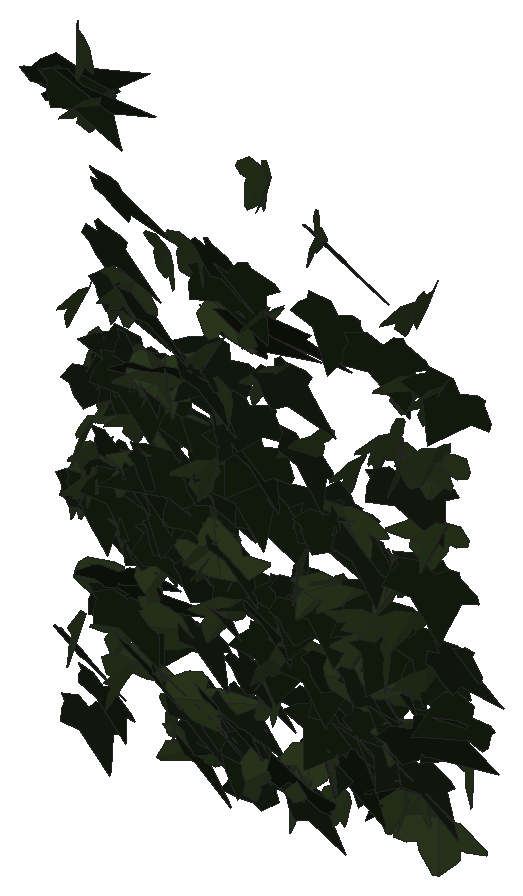
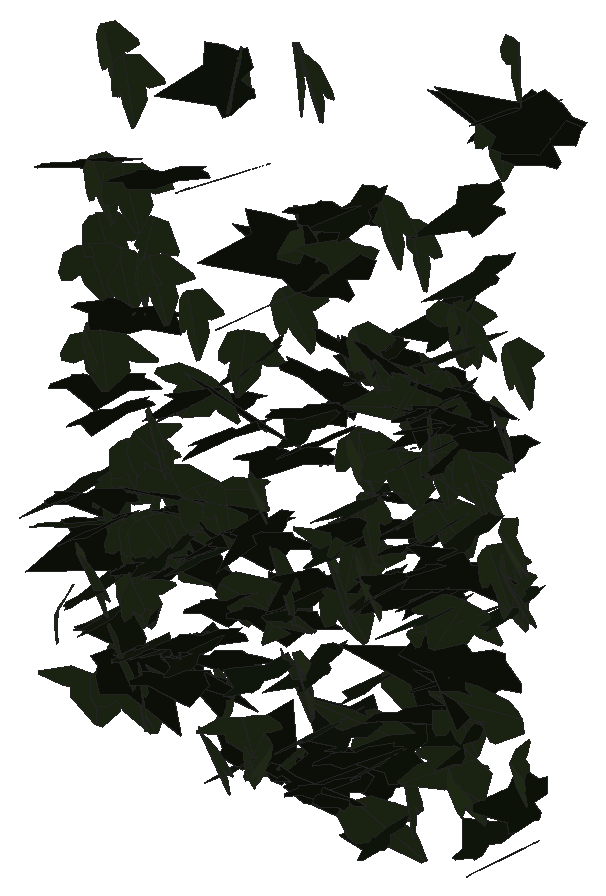
# SketchUp Ruby script. Lengths in millimetres.
U = 1.mm
M = Sketchup.active_model
def pt(a) = Geom::Point3d.new(a.map { |v| v * U })
def face(e, loops, mat)
  f = e.add_face(loops[0].map { |a| pt(a) })
  loops[1..].each { |l| e.add_face(l.map { |a| pt(a) }).erase! }
  f.material = f.back_material = mat if mat
  f
end
# faces: each face lists its corners as indices into pts; further lists are holes
def faces(e, pts, list, mat = nil) = list.each { |f| face(e, (f[0].is_a?(Array) ? f : [f]).map { |l| l.map { |i| pts[i] } }, mat) }
# xy, xz, yz: faces in a plane at the given z, y or x. An outline is a flat list of corners, or four numbers for a rectangle; further outlines are holes
def ring(l) = l.size == 4 ? [[l[0], l[1]], [l[2], l[1]], [l[2], l[3]], [l[0], l[3]]] : l.each_slice(2).to_a
def flat(e, list, mat, &to3) = list.each { |f| face(e, (f[0].is_a?(Array) ? f : [f]).map { |l| ring(l).map { |u, v| to3.(u, v) } }, mat) }
def xy(e, z, list, mat = nil) = flat(e, list, mat) { |x, y| [x, y, z] }
def xz(e, y, list, mat = nil) = flat(e, list, mat) { |x, z| [x, y, z] }
def yz(e, x, list, mat = nil) = flat(e, list, mat) { |y, z| [x, y, z] }
def lines(e, pts, list) = list.each { |a, b| e.add_line(pt(pts[a]), pt(pts[b])) }
# prism: a flat outline (further loops are holes) pulled along v
def prism(e, loops, v, mat = nil)
  f = face(e, loops, mat); d = Geom::Vector3d.new(v.map { |x| x * U })
  f.pushpull(f.normal.samedirection?(d) ? d.length : -d.length)
end
def box(e, o, s, mat = nil) = prism(e, [[o, [o[0] + s[0], o[1], o[2]], [o[0] + s[0], o[1] + s[1], o[2]], [o[0], o[1] + s[1], o[2]]]], [0, 0, s[2]], mat)
def at(x, y, z, deg = 0) = Geom::Transformation.translation(pt([x, y, z])) * Geom::Transformation.rotation(ORIGIN, Z_AXIS, deg.degrees)
def axes(o, x, y, z) = Geom::Transformation.new([*x, 0, *y, 0, *z, 0, *pt(o).to_a, 1])
def part(name) = M.definitions.add(name)
# library, detail: a bought-in or finely detailed component or shape, given as its bounding box
def library(name, o, s) = part(name).tap { |d| box(d.entities, o, s) }
def detail(e, o, s) = box(e.add_group.entities, o, s)
def put(e, d, t, mat = nil) = e.add_instance(d, t).tap { |i| i.material = mat if mat }
def group(e, t, mat = nil) = e.add_group.tap { |g| g.transformation = t; g.material = mat if mat }.entities
root = M.entities
M.materials.add("efeu1").color = [18, 25, 13]
M.materials.add("efeu2").color = [43, 57, 29]
c1 = part("ivyleaf_9")
p = [[39.1,54.8,31.7],[34.5,51.8,30.2],[-5.3,25.2,17.3],[-17.9,28.3,20.9],[-21.6,21.7,17],[-20.2,4.3,5.3],
  [-22.9,-0.3,2.5],[-17.1,-4,-0.6],[-2,-2.1,-1.2],[-0.7,-15.4,-10.1],[16.6,-22.3,-16.7],[21.1,-15.1,-12.5],
  [32.7,-10.7,-11],[46.1,-1.8,-6.6],[30.8,11.2,3.8]]
faces(c1.entities,p,[[0,1,2,3,4,5,6,7,8,9,10,11,12,13,14]],"efeu1")
c2 = part("ivyleaf_10")
p = [[0,12.8,-0.8],[-1.5,51.3,-10.9],[-4.9,51,-11.6],[-13.6,26.5,-7.3],[-13.2,15.9,-4.6],[-21.1,19.3,-7.2],
  [-29.5,16.3,-8.3],[-29.2,8.3,-6.2],[-19.7,-9.8,0.5],[-7.6,-13,4],[1,-12.2,5.8],[-0.4,51.1,-11.1],
  [-1.5,51.1,-10.9],[1,-12.4,5.9],[16.9,-12.4,3.5],[35.1,9.1,-5.1],[35,12.9,-6.1],[20.5,16.4,-4.9],
  [15.8,15,-3.8],[15.3,27.6,-7.1],[12.8,31.3,-7.8]]
faces(c2.entities,p,[[0,1,2,3,4,5,6,7,8,9,10],[11,12,0,13,14,15,16,17,18,19,20]],"efeu2")
put(root,c1,axes([1990.1,917.2,1718.9],[1.12387,-0.63107,0.1221],[0.14327,-0.09676,-0.8642],[1.21491,0.59519,-0.01104]))
put(root,c2,axes([2008.9,912.7,1745.6],[0.40299,-0.65276,0.62987],[0.55976,-0.56245,-0.68177],[1.63313,0.35386,0.07825]))
put(root,c2,axes([2015,919.8,1993.4],[0.61387,-0.7633,0.37634],[0.25359,-0.3522,-0.82855],[1.59972,0.34874,-0.01307]))
put(root,c2,axes([2011.3,925.5,1957.4],[0.80255,-0.66619,0.47453],[0.51309,-0.39084,-0.78827],[1.46967,0.50024,0.01607]))
put(root,c2,axes([2030,891.6,2498.3],[-0.97213,0.83488,0.13187],[-0.54697,-0.02666,-0.94446],[-1.51279,-0.52686,0.25675]))
put(root,c2,axes([2026.4,897.1,2176.3],[0.05785,-0.94512,0.06097],[0.02216,-0.06063,-0.94556],[1.80235,0.03108,0.00967]))
put(root,c1,axes([1991.5,894.9,2427],[0.1501,0.02213,0.98086],[1.85842,0.09385,-0.08063],[-0.18145,0.97954,-0.01443]))
put(root,c2,axes([2028,924.3,1970.1],[-0.2482,-0.88121,0.04249],[-0.01566,-0.04174,-0.89081],[1.679,-0.13066,-0.00203]))
put(root,c2,axes([2027.2,905.9,1933.9],[0.05965,-0.89479,0.23589],[0.10716,-0.23374,-0.89413],[1.75789,0.04461,0.0465]))
put(root,c2,axes([2017.5,913.4,1936.6],[1.16603,-0.58752,0.35337],[0.48398,-0.24537,-0.84885],[1.21177,0.66335,-0.00101]))
put(root,c1,axes([2008.1,914.5,1921.8],[0.66197,-0.86169,-0.09061],[-0.04948,0.08722,-0.9292],[1.64827,0.34869,0.0085]))
put(root,c1,axes([1989.1,894.6,2420.1],[0.75999,-0.14629,0.88705],[1.58589,-0.30414,-0.42527],[0.64232,0.92402,0.00046]))
put(root,c2,axes([2039.3,905.8,2111.2],[0.62311,-0.87046,-0.11063],[-0.05092,0.10813,-0.92991],[1.66921,0.32824,0.01293]))
put(root,c1,axes([2019.2,895.9,2444.3],[0.1992,-0.87795,-0.42366],[0.07153,0.42941,-0.88058],[1.8539,0.07776,0.0795]))
put(root,c2,axes([2044.4,898.7,2422.2],[-0.51083,-0.92636,-0.14907],[0.02925,0.15069,-0.96408],[1.78548,-0.2675,-0.02686]))
put(root,c1,axes([2027.1,909.1,1644.1],[0.07903,-0.88048,0.00723],[-0.00064,-0.00725,-0.88146],[1.67579,0.04152,-0.00068]))
put(root,c1,axes([2029.3,918.9,1916.4],[-0.17209,-0.89353,0.13845],[0.07065,-0.14269,-0.89667],[1.71942,-0.08357,0.0507]))
put(root,c2,axes([2020.4,924.2,1807],[-0.35173,-0.00066,-0.86106],[1.59723,-0.19716,-0.17998],[-0.36662,-0.85832,0.042]))
put(root,c1,axes([2033,927.2,1665],[0.10984,-0.76984,0.47996],[0.25295,-0.46857,-0.76755],[1.70797,0.1189,0.08281]))
put(root,c2,axes([2060,916.5,2061.2],[-0.44307,-0.89746,-0.00374],[-0.00659,0.00476,-0.92716],[1.70805,-0.23278,-0.00455]))
put(root,c1,axes([2041.2,899.1,2083.9],[0.33132,-0.44315,-0.83753],[0.01285,0.85211,-0.44946],[1.80332,0.07535,0.15708]))
put(root,c2,axes([2078.8,909.2,2200],[-1.61919,0.44371,-0.02949],[-0.18807,-0.2507,-0.92138],[-0.82517,-0.81353,0.26786]))
put(root,c1,axes([2052,898.5,2256.9],[1.02908,-0.75368,-0.2417],[-0.10045,0.25773,-0.92174],[1.503,0.53326,0.10388]))
put(root,c2,axes([2088.4,918.4,2049.3],[1.45985,0.05981,-0.52265],[-1.00038,0.04982,-0.76572],[-0.04043,0.92685,0.07488]))
put(root,c2,axes([2079.2,912.6,1708.9],[0.12496,-0.88374,0.32845],[0.03978,-0.3278,-0.88617],[1.79391,0.06883,-0.00323]))
put(root,c1,axes([2077.4,899.4,1839.3],[1.22739,0.6361,-0.27839],[-0.36762,-0.20059,-0.90581],[-1.26933,0.67318,-0.00685]))
put(root,c1,axes([2056.2,921.6,2188.5],[0.59629,-0.83809,-0.26319],[0.10399,0.29748,-0.88224],[1.66862,0.28096,0.14903]))
put(root,c1,axes([2057.7,918.5,1983.1],[0.44094,-0.90044,0.27415],[0.12071,-0.26676,-0.92975],[1.78731,0.24016,-0.00484]))
put(root,c2,axes([2085.6,901.3,2200.9],[-0.10632,-0.94317,0.10208],[0.04003,-0.10346,-0.94444],[1.80508,-0.05326,0.02696]))
put(root,c1,axes([2059.8,923.5,1952.1],[-0.45177,-0.37457,-0.79739],[1.02127,0.59349,-0.43853],[1.32977,-0.58305,0.06589]))
put(root,c1,axes([2060.2,893,2326.8],[1.43127,-0.51566,-0.29418],[-0.21832,0.33961,-0.88854],[1.10858,0.73264,0.20482]))
put(root,c2,axes([2089.7,903,1778.1],[-0.70668,-0.78897,0.20128],[-0.08513,-0.20112,-0.87086],[1.54732,-0.3714,0.04401]))
put(root,c1,axes([2080.2,917.8,1940.1],[-0.78015,-0.78959,-0.16269],[0.17537,0.13543,-0.88945],[1.52427,-0.41971,0.01906]))
put(root,c2,axes([2083.5,911.3,1890.1],[-1.60821,-0.14706,-0.20845],[0.40193,0.00133,-0.85703],[0.27234,-0.87033,0.03391]))
put(root,c1,axes([2098.9,911.3,2118.6],[-1.63713,-0.36913,-0.1268],[0.22874,0.04145,-0.93601],[0.70673,-0.8685,0.00922]))
put(root,c2,axes([2076.9,913.2,1727.6],[-0.92159,-0.27206,-0.68845],[1.16217,0.31822,-0.55526],[0.79638,-0.77921,0.01361]))
put(root,c2,axes([2105.3,907.5,1984.7],[-0.88953,-0.68114,0.40284],[-0.18018,-0.41637,-0.81385],[1.49527,-0.45538,0.14158]))
put(root,c1,axes([2080.3,911.9,1803.8],[-0.86853,-0.30959,-0.73877],[1.21639,0.37179,-0.55061],[0.91895,-0.78473,0.03059]))
put(root,c2,axes([2104.7,904.6,2052],[-0.53625,-0.95589,-0.13853],[0.07205,0.13326,-0.99655],[1.83685,-0.28429,-0.00135]))
put(root,c1,axes([2089.7,899.6,1806.1],[-0.17767,-0.79826,-0.4047],[0.1152,0.40033,-0.80361],[1.69943,-0.11059,0.01216]))
put(root,c1,axes([2093.4,920.8,2113.9],[0.08019,-0.89919,0.24159],[-0.02149,-0.24232,-0.89991],[1.7719,0.03775,-0.02185]))
put(root,c1,axes([2081.4,908.5,1747.1],[0.80924,-0.75365,0.41974],[0.38074,-0.36905,-0.8653],[1.59704,0.46987,-0.00639]))
put(root,c1,axes([2099.9,907.2,2098.7],[-0.54646,-0.94966,-0.20046],[0.14069,0.18705,-0.99198],[1.84186,-0.29604,0.0163]))
put(root,c1,axes([2127.4,917.6,2091.2],[-1.56948,-0.3673,0.14155],[-0.244,-0.06006,-0.90275],[0.70831,-0.83455,0.00267]))
put(root,c2,axes([2146.3,906.3,1791.5],[-0.60734,-0.0873,0.93419],[-1.65812,-0.33871,-0.32926],[0.66286,-0.92727,0.03232]))
put(root,c2,axes([2114.8,911.8,2094.9],[0.39495,-0.8249,-0.38584],[0.08041,0.40402,-0.84105],[1.73133,0.16941,0.12708]))
put(root,c1,axes([2099.4,919.5,1907.4],[0.14005,-0.87197,-0.23761],[-0.04436,0.23648,-0.87507],[1.71948,0.07712,-0.00322]))
put(root,c1,axes([2095.4,911.5,1888.2],[0.86165,-0.65292,-0.42802],[-0.10478,0.46685,-0.77039],[1.48215,0.41258,0.19437]))
put(root,c1,axes([2101.7,917.7,1972],[0.23204,-0.89795,0.0866],[-0.00199,-0.08752,-0.9061],[1.71691,0.12126,-0.01276]))
put(root,c1,axes([2094.5,901.3,2194.3],[1.04166,-0.78648,0.00423],[0.00467,-0.00345,-0.95818],[1.49684,0.54733,0.00004]))
put(root,c1,axes([2103.8,930.9,2061.6],[0.09179,-0.91788,-0.03431],[-0.00004,0.03436,-0.91915],[1.74814,0.0482,0.00178]))
put(root,c1,axes([2100,906.9,2080.8],[0.17781,-0.78896,-0.46319],[0.28795,0.47251,-0.77432],[1.71722,0.00246,0.1778]))
put(root,c2,axes([2124,890.9,1845.4],[0.21699,0.3029,-0.87536],[0.375,0.85385,0.32112],[1.72256,-0.22404,0.04036]))
put(root,c1,axes([2094.2,904.8,1813],[0.73125,0.39717,-0.69678],[0.93475,0.49428,0.55257],[1.20673,-0.62355,-0.0058]))
put(root,c2,axes([2099.6,903.5,2115.7],[0.98585,-0.27331,0.72979],[1.36726,-0.17212,-0.57436],[0.57476,0.87823,0.11455]))
put(root,c2,axes([2137.2,930,2038.6],[-1.42077,-0.4676,0.24131],[-0.14763,-0.31648,-0.85322],[0.99051,-0.71789,0.21897]))
put(root,c1,axes([2128.5,939.2,1777.6],[-0.85865,-0.74076,0.1948],[-0.11283,-0.19163,-0.86601],[1.45337,-0.45252,0.04786]))
put(root,c1,axes([2132.5,889.7,2119.6],[1.15059,0.69126,-0.23101],[-0.41343,-0.1156,-0.91441],[-1.32408,0.63678,0.08478]))
put(root,c1,axes([2114,910.6,1991.2],[0.71691,-0.79179,-0.36382],[-0.16361,0.36066,-0.87391],[1.65031,0.37971,0.07141]))
put(root,c2,axes([2136.4,895.2,2106.2],[-1.35078,-0.61609,-0.09163],[0.1534,0.0469,-0.93968],[1.17548,-0.71409,0.01734]))
put(root,c1,axes([2157.2,908.9,1985.5],[-1.49871,-0.13372,0.41417],[-0.64923,-0.34209,-0.75903],[0.5144,-0.82135,0.24871]))
put(root,c2,axes([2144.5,893.9,2266.7],[1.0362,-0.56301,-0.54749],[-0.20681,0.60578,-0.73101],[1.48025,0.47875,0.28113]))
put(root,c2,axes([2142.1,910.9,1681.7],[0.80547,-0.68856,-0.35026],[-0.02479,0.39296,-0.78824],[1.47007,0.3839,0.17862]))
put(root,c1,axes([2136,915.6,1945.5],[-0.56028,-0.84998,0.17314],[-0.04784,-0.1744,-0.89892],[1.65021,-0.29364,0.03273]))
put(root,c2,axes([2138.9,910.9,2110.1],[-0.21004,0.85643,-0.38111],[-0.01042,-0.38432,-0.86207],[-1.78402,-0.09859,0.0499]))
put(root,c2,axes([2130.5,894.7,2101.7],[1.00533,0.39959,-0.74001],[1.07122,0.48134,0.66168],[1.18929,-0.77134,0.02955]))
put(root,c1,axes([2133.1,907.7,1900],[-0.34938,-0.70491,-0.66266],[0.60496,0.5931,-0.71897],[1.73909,-0.34793,0.11698]))
put(root,c2,axes([2124.5,910.3,2094.4],[0.46532,0.02953,0.90419],[1.21429,0.6584,-0.19403],[-1.22066,0.66622,0.15167]))
put(root,c2,axes([2178.7,926.4,1644.7],[-0.98238,-0.33143,0.64728],[-1.0416,-0.34563,-0.61341],[0.91134,-0.7523,-0.00335]))
put(root,c1,axes([2138.7,909.2,1908.4],[0.48819,-0.85582,-0.15606],[-0.03607,0.15717,-0.89304],[1.65527,0.25583,0.02656]))
put(root,c1,axes([2139.7,911.8,1719.4],[1.33092,-0.59191,0.15775],[0.25536,-0.08559,-0.91594],[1.13753,0.71175,0.02104]))
put(root,c1,axes([2149.6,932.8,1636],[0.69173,-0.77962,0.17603],[0.09501,-0.17085,-0.85978],[1.51816,0.36592,-0.0264]))
put(root,c2,axes([2179.5,895.9,2280.9],[1.1931,-0.55168,-0.48414],[-0.26301,0.53659,-0.79038],[1.37195,0.58263,0.2695]))
put(root,c1,axes([2161.9,914.8,1707],[0.40723,-0.90516,-0.07843],[-0.01788,0.07836,-0.93006],[1.72906,0.21399,0.00885]))
put(root,c2,axes([2186.5,925.5,2149.9],[-0.07398,-0.91971,0.09255],[-0.01583,-0.09228,-0.92052],[1.75916,-0.03951,-0.00439]))
put(root,c2,axes([2189.6,913,1965.6],[0.90977,-0.39709,-0.68129],[-0.32278,0.72628,-0.54231],[1.46568,0.40642,0.30346]))
put(root,c1,axes([2181.5,939.4,2031.5],[-0.79442,-0.73143,0.3281],[-0.00202,-0.36941,-0.82487],[1.52569,-0.38134,0.16975]))
put(root,c1,axes([2168.9,926.6,1788.9],[0.29893,-0.85192,0.05262],[0.02886,-0.05071,-0.86626],[1.6242,0.15769,0.00571]))
put(root,c1,axes([2206.9,926.4,2140.9],[-1.74286,-0.06933,-0.13389],[0.25268,0.01984,-0.91832],[0.13601,-0.92527,-0.00965]))
put(root,c1,axes([2186.2,933.8,1711.2],[-0.532,-0.84061,-0.04696],[0.03055,0.04415,-0.88587],[1.60205,-0.27999,0.0013]))
put(root,c2,axes([2197.1,908.4,1895.5],[0.30325,-0.912,-0.03122],[-0.01071,0.03071,-0.92582],[1.73671,0.15944,-0.00026]))
put(root,c1,axes([2173.4,923.5,1984.7],[0.76561,-0.78659,-0.26275],[-0.02561,0.2858,-0.8762],[1.57814,0.38624,0.11325]))
put(root,c1,axes([2180,919.3,1952.6],[-0.3621,-0.8046,-0.46367],[0.29687,0.43889,-0.8256],[1.74228,-0.242,0.04431]))
put(root,c1,axes([2176.8,910.8,2125.5],[0.51713,-0.86241,0.24413],[0.19338,-0.22382,-0.90375],[1.69485,0.28868,0.02863]))
put(root,c1,axes([2181.4,900.8,1876.7],[0.80291,-0.80198,-0.26254],[-0.23026,0.233,-0.90617],[1.58944,0.43888,0.00135]))
put(root,c2,axes([2206,899.9,2018.8],[-0.76166,-0.8357,0.05175],[0.03132,-0.06519,-0.92559],[1.59324,-0.39823,0.04294]))
put(root,c2,axes([2207.1,906.4,2019.6],[0.20545,-0.88337,0.26344],[0.11945,-0.25759,-0.88944],[1.75032,0.12127,0.02978]))
put(root,c2,axes([2209.4,903.7,1917.2],[-0.61526,-0.81143,-0.36202],[0.2962,0.32757,-0.87319],[1.6649,-0.35814,0.02157]))
put(root,c2,axes([2174.2,898.1,1716.7],[0.59568,-0.06197,-0.93896],[1.78754,0.08135,0.30771],[0.10999,-0.98641,0.08437]))
put(root,c2,axes([2217.6,924.8,1886.9],[0.66766,-0.82354,-0.15066],[-0.0494,0.15257,-0.89445],[1.59261,0.34998,0.03542]))
put(root,c1,axes([2193.8,911.2,2281.3],[0.98116,-0.8013,-0.06183],[-0.0663,0.05111,-0.95281],[1.52812,0.51671,-0.00164]))
put(root,c2,axes([2222.7,900.5,2111.6],[1.02812,-0.71716,-0.28043],[-0.1085,0.30437,-0.8882],[1.46152,0.52709,0.13133]))
put(root,c2,axes([2229.3,900.8,1849.5],[-0.59875,-0.83352,0.29326],[-0.05523,-0.30138,-0.88773],[1.68077,-0.30683,0.0753]))
put(root,c2,axes([2220.2,895.7,1900.8],[1.74589,0.41204,0.03032],[-0.05323,-0.01174,1.00563],[0.78451,-0.91777,0.00075]))
put(root,c1,axes([2201.6,914.1,1683.8],[-0.20323,-0.31698,-0.8491],[1.05928,0.65184,-0.31334],[1.36138,-0.55451,0.11705]))
put(root,c1,axes([2224.4,933.5,1663.1],[-0.60702,-0.78923,-0.00888],[0.0101,0.00744,-0.85124],[1.50213,-0.31899,0.00213]))
put(root,c1,axes([2204.6,925.6,1661.7],[0.45959,-0.51982,0.65489],[0.59985,-0.57478,-0.57245],[1.47391,0.39601,0.02877]))
put(root,c1,axes([2239.5,921.6,2094.9],[-1.56006,-0.29686,-0.29948],[0.54024,0.09567,-0.87178],[0.59348,-0.86744,0.00634]))
put(root,c1,axes([2216.3,919,1915.4],[0.28207,-0.86585,0.24442],[0.14999,-0.23426,-0.87767],[1.7057,0.16378,0.03676]))
put(root,c2,axes([2221.6,898.9,2221.7],[0.71236,0.81601,0.44998],[0.35784,0.40882,-0.89775],[-1.73703,0.41886,-0.0004]))
put(root,c1,axes([2213.7,911.2,1711.1],[0.24922,-0.72975,0.60412],[0.59379,-0.54262,-0.72309],[1.70243,0.29609,0.16377]))
put(root,c1,axes([2223,917.4,1723.5],[0.72962,-0.70979,-0.38475],[-0.13159,0.39549,-0.7985],[1.53093,0.37227,0.11473]))
put(root,c1,axes([2229.2,902.2,2267],[-0.33272,-0.77669,-0.51982],[0.41333,0.4806,-0.79113],[1.73002,-0.2642,0.08904]))
put(root,c1,axes([2281,913.7,1635],[-1.46981,-0.07686,-0.43448],[-0.82271,-0.04373,0.7761],[-0.16829,0.88503,0.00061]))
put(root,c1,axes([2258.4,921.9,2050],[-1.10834,-0.70616,0.17703],[-0.10534,-0.1831,-0.91244],[1.38153,-0.58047,0.07245]))
put(root,c1,axes([2238.3,918.5,1874.9],[-0.06237,-0.66263,-0.62972],[0.246,0.62043,-0.65959],[1.72228,-0.11262,0.0714]))
put(root,c2,axes([2264.7,920,1770.1],[0.35253,-0.80556,-0.24121],[-0.12138,0.23282,-0.82653],[1.59579,0.19567,-0.00958]))
put(root,c1,axes([2241.9,911.6,1776.9],[0.97876,-0.76823,-0.21215],[-0.17105,0.19497,-0.92389],[1.50714,0.52102,0.03292]))
put(root,c1,axes([2246.4,926.6,2035.5],[0.21942,-0.80126,0.42132],[0.19286,-0.41063,-0.80866],[1.7121,0.14894,0.0371]))
put(root,c1,axes([2227,905.4,2197.8],[0.77821,-0.27682,0.82119],[1.39736,-0.37168,-0.49088],[0.87613,0.83869,0.0535]))
put(root,c1,axes([2253.7,905.5,2011.2],[-0.09384,-0.92681,0.00081],[0.00444,-0.00093,-0.92812],[1.7639,-0.0493,0.00238]))
put(root,c2,axes([2265.9,894.2,2212.8],[0.43559,-0.22668,0.96193],[-0.29585,0.96684,0.26482],[-1.85748,-0.20715,0.1834]))
put(root,c2,axes([2270.2,900.3,2406],[1.15271,-0.73019,-0.20182],[-0.03604,0.24371,-0.93861],[1.44135,0.59006,0.13793]))
put(root,c2,axes([2279.9,917.5,2155.6],[-0.2686,-0.90335,0.18428],[-0.09334,-0.1788,-0.91408],[1.75218,-0.148,-0.02045]))
put(root,c2,axes([2284.5,897.4,2407.5],[0.50566,-0.83161,-0.43011],[0.00363,0.44757,-0.8642],[1.78188,0.23508,0.12382]))
put(root,c2,axes([2287,905.7,1755.6],[0.92506,-0.70274,-0.28183],[-0.23348,0.25739,-0.85336],[1.42196,0.49943,0.04323]))
put(root,c2,axes([2277.1,879.8,1661.3],[0.1456,-0.10269,-0.94407],[0.52944,0.908,-0.07622],[1.72806,-0.26954,0.1029]))
put(root,c1,axes([2265.8,923.6,1836.8],[0.09928,-0.67786,0.55598],[0.3522,-0.5359,-0.67074],[1.63094,0.15699,0.111]))
put(root,c2,axes([2297.2,911.5,1865.6],[0.90225,-0.73454,-0.50008],[-0.27797,0.49468,-0.86507],[1.66821,0.4797,0.12632]))
put(root,c1,axes([2295.3,919.8,1816.3],[-1.06655,-0.68176,-0.20575],[0.26093,0.15363,-0.88249],[1.32998,-0.57687,0.00814]))
put(root,c1,axes([2266.8,916.1,2213.4],[1.68326,-0.09046,0.31445],[0.59541,-0.03169,-0.88905],[0.18242,0.93814,0.00029]))
put(root,c1,axes([2283.9,913.5,1991.1],[-0.27526,-0.80789,-0.42978],[0.29065,0.4077,-0.81778],[1.71718,-0.19851,0.06952]))
put(root,c2,axes([2303.1,885.9,1814.9],[-0.39803,-0.61059,-0.74498],[0.39746,0.71546,-0.64502],[1.78962,-0.2947,-0.02244]))
put(root,c1,axes([2287.8,915.3,2156.5],[0.68846,-0.74749,-0.4514],[-0.0611,0.47689,-0.81542],[1.66078,0.32741,0.15713]))
put(root,c2,axes([2342.2,913,1819.7],[0.44886,0.0086,-0.88225],[-1.61416,0.25387,-0.22425],[0.46273,0.87723,0.07355]))
put(root,c2,axes([2309.2,920.4,1663.8],[-0.73552,0.73817,-0.21038],[0.17896,-0.18824,-0.83321],[-1.44983,-0.39772,0.00389]))
put(root,c1,axes([2298.4,934.2,1751],[0.27693,-0.82173,0.2304],[0.29893,-0.20395,-0.82658],[1.59648,0.18073,0.11481]))
put(root,c1,axes([2321.4,908.1,1642.7],[1.27753,-0.44023,0.40048],[-0.63621,0.22055,0.80274],[-0.93711,-0.74988,0.00098]))
put(root,c1,axes([2312.3,912.4,1907.2],[0.34464,-0.52398,-0.70922],[-0.47028,0.66485,-0.5543],[1.61097,0.30619,-0.01009]))
put(root,c1,axes([2325.2,916.7,1886.2],[-1.06057,-0.73513,-0.12476],[0.10837,0.11335,-0.92218],[1.41496,-0.55969,-0.02289]))
put(root,c2,axes([2334.3,915.4,2090.4],[-0.60032,-0.8219,-0.31637],[0.19709,0.29911,-0.88029],[1.66449,-0.33184,-0.00987]))
put(root,c2,axes([2330.2,924.2,1688],[1.0895,0.61048,-0.20411],[-0.22531,-0.16864,-0.83642],[-1.20419,0.58389,-0.02817]))
put(root,c2,axes([2326.7,909.7,1938],[0.55356,-0.66861,0.59019],[0.57654,-0.5098,-0.72684],[1.59641,0.41596,0.05785]))
put(root,c2,axes([2330.5,908.8,1649.8],[0.09534,-0.70202,0.61785],[0.46339,-0.58761,-0.6874],[1.71846,0.1974,0.15108]))
put(root,c1,axes([2324.5,917.8,2073.7],[0.16363,-0.89241,0.28531],[0.00269,-0.28638,-0.8962],[1.78312,0.08233,-0.02483]))
put(root,c1,axes([2375,901.9,2011.9],[-0.53646,0.57149,0.64541],[-1.04473,0.40459,-0.59799],[-1.26506,-0.57647,0.22015]))
put(root,c1,axes([2328.9,907.8,1646.2],[0.6031,-0.74652,-0.26021],[-0.12873,0.25371,-0.81023],[1.49909,0.32212,0.03511]))
put(root,c1,axes([2329.8,897.1,1890.9],[0.71322,-0.6045,-0.70261],[-0.0948,0.74364,-0.66637],[1.76147,0.28479,0.24863]))
put(root,c2,axes([2357.6,913.3,1917.6],[-0.58343,-0.82735,-0.13894],[0.05403,0.13762,-0.88207],[1.59575,-0.30715,-0.02094]))
put(root,c2,axes([2358.9,910.1,1917.9],[-0.45438,-0.63954,0.58],[-0.02597,-0.59889,-0.666],[1.64296,-0.18634,0.14988]))
put(root,c1,axes([2353,919,1809.4],[-0.59346,-0.81495,-0.1063],[0.02136,0.10946,-0.87211],[1.56401,-0.31073,-0.02843]))
put(root,c2,axes([2362.7,886.7,2370.5],[0.22925,-0.59248,-0.75944],[0.10155,0.76828,-0.59091],[1.83037,0.03158,0.1279]))
put(root,c1,axes([2343.6,920,1997],[0.29038,-0.82717,-0.39116],[0.02466,0.39847,-0.83759],[1.74125,0.1323,0.07709]))
put(root,c1,axes([2371.2,919.8,1744.2],[-1.17531,-0.60535,0.08134],[-0.05832,-0.08481,-0.86388],[1.16098,-0.61708,0.03894]))
put(root,c2,axes([2357.5,915,1705.1],[-0.54469,0.50806,-0.64258],[0.34686,-0.62412,-0.57463],[-1.51996,-0.32449,0.09914]))
put(root,c2,axes([2372.7,920.8,1647.2],[0.97943,-0.67349,-0.09226],[-0.10537,0.0738,-0.84759],[1.28945,0.51759,0.00081]))
put(root,c2,axes([2381.5,919.7,1908.4],[-0.7171,-0.72651,0.42423],[-0.13322,-0.43615,-0.80909],[1.5956,-0.36292,0.1231]))
put(root,c1,axes([2369.7,917.1,2255.8],[-0.53032,-0.85434,0.28727],[0.00869,-0.30202,-0.89377],[1.71541,-0.26259,0.09334]))
put(root,c1,axes([2372.3,912.4,1898.2],[-1.05545,-0.67028,-0.3031],[0.39651,0.22093,-0.86976],[1.34272,-0.59212,0.01859]))
put(root,c1,axes([2369.1,936.2,1856.1],[-0.11175,-0.86578,0.26803],[0.06406,-0.27049,-0.86636],[1.72372,-0.04608,0.04958]))
put(root,c1,axes([2356.8,899.5,2360.7],[1.52586,-0.54579,0.07032],[0.0988,-0.0487,-0.96981],[1.04267,0.80333,-0.01102]))
put(root,c1,axes([2382.9,923.8,1723.2],[-1.35684,-0.22437,-0.44965],[0.89156,-0.01429,-0.73562],[0.34611,-0.84276,0.13218]))
put(root,c1,axes([2375.5,930,1767.9],[-0.3235,-0.82115,-0.27496],[0.07619,0.27246,-0.83842],[1.64633,-0.17396,-0.01523]))
put(root,c1,axes([2377.8,933.7,1749.8],[0.48611,-0.79521,0.25974],[0.17284,-0.24362,-0.83515],[1.58273,0.27084,0.01143]))
put(root,c1,axes([2377.3,898.3,2013.7],[0.25663,-0.69,-0.66873],[0.37846,0.6807,-0.66226],[1.78917,-0.04502,0.23601]))
put(root,c2,axes([2395.7,904.5,2020.8],[-1.62921,0.16176,-0.25789],[0.39136,-0.2603,-0.84583],[-0.42723,-0.85531,0.20864]))
put(root,c1,axes([2373.9,904.5,1832],[-0.05302,-0.27695,-0.87625],[1.62147,0.32083,-0.12849],[0.65561,-0.81588,0.24692]))
put(root,c1,axes([2406.5,934.5,1716.2],[-0.95416,-0.70507,-0.10785],[0.08723,0.09971,-0.86491],[1.3547,-0.50303,-0.02027]))
put(root,c2,axes([2411.8,898,2097.6],[-0.10137,-0.93016,-0.17136],[0.07946,0.16915,-0.93115],[1.79831,-0.05991,0.03149]))
put(root,c2,axes([2416.5,904.7,1869.2],[-0.31287,-0.83355,0.36866],[0.08945,-0.38186,-0.84244],[1.73233,-0.13083,0.11008]))
put(root,c1,axes([2426.8,936.6,1907.6],[-1.51198,-0.38878,0.17348],[-0.03939,-0.33158,-0.83786],[0.80929,-0.74249,0.28333]))
put(root,c1,axes([2395.8,904.1,1711.5],[-0.51314,-0.00969,-0.84737],[1.60703,0.0723,-0.2695],[0.1367,-0.88629,-0.01272]))
put(root,c2,axes([2435.8,899.6,1903.2],[-1.31759,-0.54025,0.31172],[-0.44626,-0.20611,-0.87799],[1.10001,-0.73073,0.01719]))
put(root,c1,axes([2415.6,933.1,1746.6],[-0.38519,-0.82196,0.17649],[-0.05479,-0.17465,-0.84641],[1.59908,-0.20398,0.01351]))
put(root,c2,axes([2433.5,930.6,1863.4],[-0.73545,-0.69108,0.39779],[-0.13157,-0.41134,-0.78178],[1.51188,-0.37197,0.12547]))
put(root,c1,axes([2416.2,910.2,1989.1],[-0.07414,-0.91158,0.17875],[-0.00937,-0.17871,-0.91241],[1.76794,-0.03917,0.00266]))
put(root,c2,axes([2394.7,895,1821.4],[0.4268,-0.15758,-0.89109],[1.62806,-0.2625,0.2617],[-0.56169,-0.88058,0.08145]))
put(root,c1,axes([2417.6,902.4,1829.3],[0.7244,-0.84013,-0.35561],[-0.15505,0.35248,-0.91993],[1.72933,0.38352,0.06648]))
put(root,c2,axes([2443,914.6,2130.9],[-0.31048,-0.93617,-0.03922],[0.01799,0.03816,-0.95027],[1.78319,-0.16338,0.00276]))
put(root,c1,axes([2416.6,931.8,1842.8],[0.50457,-0.82556,0.2728],[0.21983,-0.24923,-0.86649],[1.6401,0.28739,0.03221]))
put(root,c2,axes([2443.3,917.5,1966.7],[0.69269,-0.77059,-0.31438],[-0.11027,0.31884,-0.84858],[1.58009,0.36006,0.0786]))
put(root,c2,axes([2448.4,929.7,1860.3],[-0.57122,-0.76011,0.36353],[-0.0497,-0.37733,-0.81052],[1.6028,-0.28259,0.10442]))
put(root,c1,axes([2438.7,921.9,1821],[-0.69264,-0.83749,-0.02495],[0.01738,0.02324,-0.91315],[1.59453,-0.36405,-0.00088]))
put(root,c2,axes([2447.2,926.2,1950.9],[-0.30634,-0.71974,0.56052],[0.15681,-0.57832,-0.71894],[1.72911,-0.07507,0.16451]))
put(root,c1,axes([2434.9,917.1,2240.8],[-0.32443,-0.87063,-0.31313],[0.25189,0.29218,-0.88443],[1.74278,-0.2043,0.06954]))
put(root,c1,axes([2451.1,915.1,1868.9],[-0.94218,-0.70564,0.21497],[-0.03642,-0.24653,-0.85327],[1.40343,-0.48012,0.12218]))
put(root,c1,axes([2451.3,930.2,1722.1],[-0.77562,-0.58007,0.50539],[-0.03845,-0.56365,-0.66322],[1.46372,-0.32218,0.25038]))
put(root,c1,axes([2471,914.8,1701.7],[-0.00061,0.72675,-0.57082],[-0.01866,-0.5708,-0.7267],[-1.75869,0.00581,0.00791]))
put(root,c2,axes([2447.5,908.4,1870.1],[0.32892,-0.51553,0.74616],[0.84874,-0.61311,-0.5269],[1.50299,0.45904,0.13425]))
put(root,c2,axes([2475.8,919.1,1681.9],[-1.23245,-0.66757,0.33135],[-0.36539,-0.27473,-0.92868],[1.37054,-0.67355,0.05038]))
put(root,c2,axes([2470.4,906.9,1683.2],[0.53859,-0.69072,-0.55775],[-0.20783,0.55387,-0.74132],[1.67682,0.2905,0.08727]))
put(root,c2,axes([2467.1,910.6,1775.5],[-0.39474,-0.77307,0.34276],[0.23273,-0.37663,-0.77545],[1.59251,-0.13658,0.19829]))
put(root,c2,axes([2472.5,909.7,1836.4],[-0.80799,-0.77265,-0.09329],[0.06993,0.08625,-0.88156],[1.47954,-0.42603,-0.00928]))
put(root,c2,axes([2467.7,887,2153],[-0.15852,-0.81917,-0.55725],[0.31993,0.53942,-0.81809],[1.85824,-0.16275,0.09331]))
put(root,c2,axes([2477.3,905.2,1920.1],[-0.66068,-0.81372,0.16705],[-0.06852,-0.16614,-0.88411],[1.57948,-0.34758,0.03152]))
put(root,c2,axes([2479.6,912,2216.2],[-0.62094,-0.89624,0.01194],[-0.0069,-0.01139,-0.95378],[1.70586,-0.32628,0.00049]))
put(root,c2,axes([2477.6,888.2,2120.4],[0.42674,-0.76891,-0.52224],[-0.02096,0.53498,-0.79241],[1.76889,0.19184,0.1166]))
put(root,c2,axes([2479.3,904,1784.2],[-0.24835,-0.88511,-0.01911],[0.00191,0.01917,-0.89468],[1.68494,-0.13048,-0.0018]))
put(root,c2,axes([2494.9,909.2,2122.5],[-1.62281,0.1476,0.327],[-0.63593,-0.01969,-0.8624],[-0.24864,-0.91302,0.07147]))
put(root,c1,axes([2467.4,919.9,2083.4],[-0.54364,-0.64315,-0.59252],[0.5236,0.52558,-0.70313],[1.57981,-0.39551,0.02914]))
put(root,c2,axes([2490.2,896.3,2322],[-0.2537,-0.94983,-0.2069],[0.05017,0.20523,-0.95914],[1.84943,-0.13586,-0.00236]))
put(root,c1,axes([2468.8,907,1734.4],[0.95536,-0.68368,0.19339],[0.22628,-0.15261,-0.84816],[1.33317,0.51584,0.00538]))
put(root,c1,axes([2483.1,930.7,1974.4],[-0.17123,-0.9049,-0.15923],[-0.02213,0.1611,-0.90896],[1.74853,-0.08657,-0.0271]))
put(root,c2,axes([2479.1,922.5,1706.8],[0.83124,-0.48327,0.57608],[0.96004,-0.30574,-0.63893],[1.06129,0.65509,0.12678]))
put(root,c2,axes([2503.4,920.3,2033.9],[-1.31568,-0.62824,0.08275],[0.12077,-0.19049,-0.91603],[1.19994,-0.66967,0.18293]))
put(root,c2,axes([2509.7,893.7,1866.2],[-0.42658,-0.85782,-0.22933],[0.14889,0.21653,-0.88639],[1.68337,-0.23653,0.02028]))
put(root,c1,axes([2508.1,935.1,1876.8],[-1.02769,-0.72459,-0.00878],[0.00973,0.00714,-0.90366],[1.3791,-0.54001,-0.00017]))
put(root,c1,axes([2496.6,935.2,1845.3],[-0.12899,-0.89999,0.09564],[-0.03141,-0.09467,-0.90249],[1.72222,-0.06914,-0.00929]))
put(root,c2,axes([2514.1,920.2,2123.7],[-1.08174,-0.69906,0.22096],[0.02398,-0.28886,-0.88146],[1.39512,-0.53706,0.18648]))
put(root,c2,axes([2513.1,912.6,2213.9],[-0.10146,-0.95011,-0.00492],[0.0048,0.00479,-0.9516],[1.80826,-0.05332,0.00225]))
put(root,c1,axes([2507.3,938.8,1768.6],[-0.54357,-0.5158,0.68147],[-0.24605,-0.68418,-0.57203],[1.60789,-0.27907,0.14284]))
put(root,c2,axes([2517.7,899.5,2144.4],[-0.47607,-0.92495,0.04703],[-0.01663,-0.04636,-0.95817],[1.76256,-0.25027,0.00366]))
put(root,c2,axes([2516.1,893.4,2345.4],[0.04985,-0.97942,-0.10575],[0.01174,0.10595,-0.97973],[1.87482,0.02538,0.00895]))
put(root,c2,axes([2514.8,928,1794.5],[1.02742,-0.78008,-0.0211],[-0.02453,0.01674,-0.94865],[1.48498,0.53999,-0.00107]))
put(root,c2,axes([2514.7,914.7,2037],[-0.00096,-0.83337,0.44396],[0.21849,-0.44072,-0.82716],[1.78376,0.05353,0.10155]))
put(root,c1,axes([2498.8,903.4,1739.2],[0.43837,-0.93145,-0.06282],[-0.02363,0.06165,-0.9595],[1.77661,0.23065,0.00274]))
put(root,c2,axes([2512.2,913.6,1661.8],[1.80457,0.28216,0.07054],[0.11828,0.03843,-0.98908],[-0.54075,0.95002,0.01905]))
put(root,c1,axes([2516,905.4,1984.8],[-0.72948,-0.82169,-0.24492],[0.19629,0.22214,-0.90669],[1.61998,-0.39692,-0.00043]))
put(root,c1,axes([2511.4,879.3,1801.6],[-0.03888,-0.10693,-0.99921],[0.4765,0.96736,-0.10864],[1.85224,-0.2511,0.00698]))
put(root,c1,axes([2516.9,918.7,1880.2],[1.00506,-0.54388,-0.48464],[-0.27053,0.51015,-0.72739],[1.35978,0.50349,0.21349]))
put(root,c1,axes([2537.7,918.3,2217],[-1.02595,-0.73004,0.21783],[-0.00034,-0.26672,-0.89435],[1.44995,-0.51662,0.15392]))
put(root,c1,axes([2557.3,915,1817.9],[-1.22776,-0.36134,0.48606],[-0.31801,-0.57639,-0.65026],[1.10795,-0.56585,0.35198]))
put(root,c2,axes([2539.3,939.5,1736.6],[-0.02685,-0.38893,0.80756],[0.94036,-0.67724,-0.31753],[1.42332,0.4401,0.22502]))
